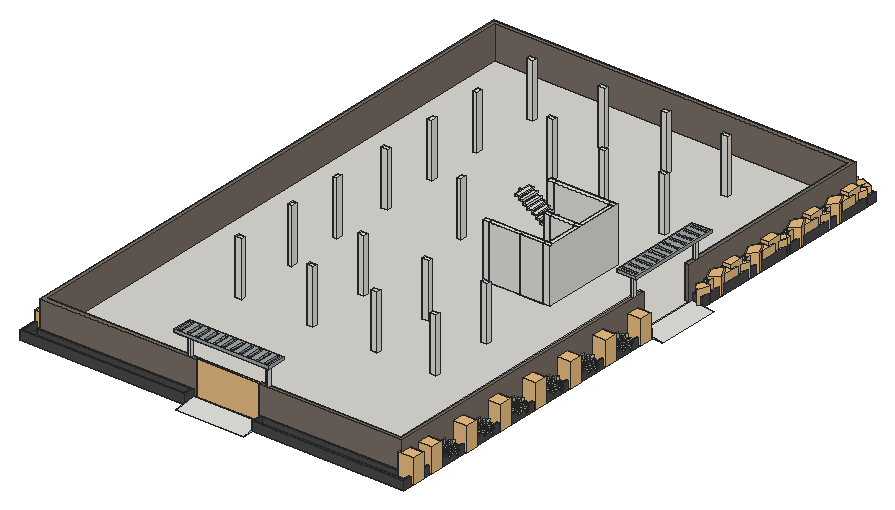
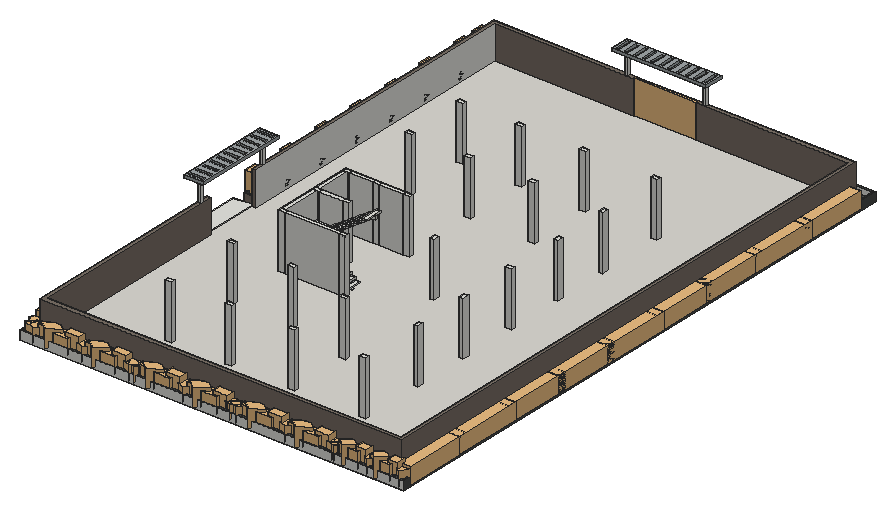
# SketchUp Ruby script. Lengths in inches.
U = 1.inch
M = Sketchup.active_model
def pt(a) = Geom::Point3d.new(a.map { |v| v * U })
def face(e, loops, mat)
  f = e.add_face(loops[0].map { |a| pt(a) })
  loops[1..].each { |l| e.add_face(l.map { |a| pt(a) }).erase! }
  f.material = f.back_material = mat if mat
  f
end
# faces: each face lists its corners as indices into pts; further lists are holes
def faces(e, pts, list, mat = nil) = list.each { |f| face(e, (f[0].is_a?(Array) ? f : [f]).map { |l| l.map { |i| pts[i] } }, mat) }
# xy, xz, yz: faces in a plane at the given z, y or x. An outline is a flat list of corners, or four numbers for a rectangle; further outlines are holes
def ring(l) = l.size == 4 ? [[l[0], l[1]], [l[2], l[1]], [l[2], l[3]], [l[0], l[3]]] : l.each_slice(2).to_a
def flat(e, list, mat, &to3) = list.each { |f| face(e, (f[0].is_a?(Array) ? f : [f]).map { |l| ring(l).map { |u, v| to3.(u, v) } }, mat) }
def xy(e, z, list, mat = nil) = flat(e, list, mat) { |x, y| [x, y, z] }
def xz(e, y, list, mat = nil) = flat(e, list, mat) { |x, z| [x, y, z] }
def yz(e, x, list, mat = nil) = flat(e, list, mat) { |y, z| [x, y, z] }
def lines(e, pts, list) = list.each { |a, b| e.add_line(pt(pts[a]), pt(pts[b])) }
# prism: a flat outline (further loops are holes) pulled along v
def prism(e, loops, v, mat = nil)
  f = face(e, loops, mat); d = Geom::Vector3d.new(v.map { |x| x * U })
  f.pushpull(f.normal.samedirection?(d) ? d.length : -d.length)
end
def box(e, o, s, mat = nil) = prism(e, [[o, [o[0] + s[0], o[1], o[2]], [o[0] + s[0], o[1] + s[1], o[2]], [o[0], o[1] + s[1], o[2]]]], [0, 0, s[2]], mat)
def at(x, y, z, deg = 0) = Geom::Transformation.translation(pt([x, y, z])) * Geom::Transformation.rotation(ORIGIN, Z_AXIS, deg.degrees)
def axes(o, x, y, z) = Geom::Transformation.new([*x, 0, *y, 0, *z, 0, *pt(o).to_a, 1])
def part(name) = M.definitions.add(name)
# library, detail: a bought-in or finely detailed component or shape, given as its bounding box
def library(name, o, s) = part(name).tap { |d| box(d.entities, o, s) }
def detail(e, o, s) = box(e.add_group.entities, o, s)
def put(e, d, t, mat = nil) = e.add_instance(d, t).tap { |i| i.material = mat if mat }
def group(e, t, mat = nil) = e.add_group.tap { |g| g.transformation = t; g.material = mat if mat }.entities
root = M.entities
M.materials.add("1484 AP 8289 COLD FLINT").color = [159, 165, 167]
M.materials.add("1488 AP 8285 MINESHAFT").color = [72, 74, 72]
M.materials.add("1495 AP 8294 DARK SHADOW").color = [102, 101, 98]
M.materials.add("Material__3").color = [95, 70, 46]
M.materials.add("StoneBricksSplitface001_4K").color = [121, 111, 102]
M.materials.add("[Terrazzo Tile Light]").color = [219, 217, 210]
M.materials.add("hymenocallis littoralis").color = [156, 172, 146]
c1 = part("1")
box(c1.entities,[0,0,0],[14,9,117])
c2 = part("Group\#131")
box(c2.entities,[0,0,0],[6,6,48])
c3 = library("Group\#239",[0,0,-0.25],[37,199,0.25])
c4 = part("21")
put(c4.entities,c2,at(18,15,0))
g1 = group(c4.entities,at(18,12,48),"1484 AP 8289 COLD FLINT")
xy(g1,0,[[-18,-12,24,192]],"1484 AP 8289 COLD FLINT")
xy(g1,6,[[[-18,-12,24,192],[-12,-6,18,0],[-12,12.6,18,18.6],[-12,31.2,18,37.2],[-12,49.8,18,55.8],[-12,68.4,18,74.4],[-12,87,18,93],[-12,105.6,18,111.6],[-12,124.2,18,130.2],[-12,142.8,18,148.8],[-12,161.4,18,167.4],[-12,180,18,186]]])
xz(g1,-12,[[-18,0,24,6]],"1484 AP 8289 COLD FLINT")
xz(g1,-6,[[-12,0,18,6]])
xz(g1,0,[[-12,0,18,6]])
xz(g1,12.6,[[-12,0,18,6]])
xz(g1,18.6,[[-12,0,18,6]])
xz(g1,31.2,[[-12,0,18,6]])
xz(g1,37.2,[[-12,0,18,6]])
xz(g1,49.8,[[-12,0,18,6]])
xz(g1,55.8,[[-12,0,18,6]])
xz(g1,68.4,[[-12,0,18,6]])
xz(g1,74.4,[[-12,0,18,6]])
xz(g1,87,[[-12,0,18,6]])
xz(g1,93,[[-12,0,18,6]])
xz(g1,105.6,[[-12,0,18,6]])
xz(g1,111.6,[[-12,0,18,6]])
xz(g1,124.2,[[-12,0,18,6]])
xz(g1,130.2,[[-12,0,18,6]])
xz(g1,142.8,[[-12,0,18,6]])
xz(g1,148.8,[[-12,0,18,6]])
xz(g1,161.4,[[-12,0,18,6]])
xz(g1,167.4,[[-12,0,18,6]])
xz(g1,180,[[-12,0,18,6]])
xz(g1,186,[[-12,0,18,6]])
xz(g1,192,[[-18,0,24,6]])
yz(g1,-18,[[-12,0,192,6]],"1484 AP 8289 COLD FLINT")
yz(g1,-12,[[-6,0,0,6],[12.6,0,18.6,6],[31.2,0,37.2,6],[49.8,0,55.8,6],[68.4,0,74.4,6],
  [87,0,93,6],[105.6,0,111.6,6],[124.2,0,130.2,6],[142.8,0,148.8,6],[161.4,0,167.4,6],
  [180,0,186,6]])
yz(g1,18,[[-6,0,0,6],[12.6,0,18.6,6],[31.2,0,37.2,6],[49.8,0,55.8,6],[68.4,0,74.4,6],
  [87,0,93,6],[105.6,0,111.6,6],[124.2,0,130.2,6],[142.8,0,148.8,6],[161.4,0,167.4,6],
  [180,0,186,6]])
yz(g1,24,[[-12,0,192,6]])
put(g1,c3,at(-15.5,-9.5,0))
g2 = group(g1,at(22,-10,0),"1495 AP 8294 DARK SHADOW")
xy(g2,-0.5,[[[-38,0,0,200],[-37.5,0.5,-0.5,199.5]]])
xz(g2,0,[[-38,-0.5,0,0]])
xz(g2,0.5,[[-37.5,-0.5,-0.5,0]])
xz(g2,199.5,[[-37.5,-0.5,-0.5,0]])
xz(g2,200,[[-38,-0.5,0,0]])
yz(g2,-38,[[0,-0.5,200,0]])
yz(g2,-37.5,[[0.5,-0.5,199.5,0]])
yz(g2,-0.5,[[0.5,-0.5,199.5,0]])
yz(g2,0,[[0,-0.5,200,0]])
put(c4.entities,c2,axes([18,189,0],[1,0,0],[0,-1,0],[0,0,1]))
c5 = library("Gate_Lasercut_10ftx6ft_Kalil",[-0.15,-3.25,-0.15],[120,5.625,60.3])
c6 = part("90")
box(c6.entities,[0,-39,3],[11,39,3])
c7 = part("Group\#94")
box(c7.entities,[-50,0,0],[50,9,117])
c8 = part("Group\#856")
xy(c8.entities,7.38,[[0,0,5.5,15.91]],"hymenocallis littoralis")
p = [[5.5,28.78,0],[5.5,26.79,3.44],[0,26.79,3.44],[0,28.78,0],[0,23.75,6],[5.5,23.75,6],
  [0,15.91,7.38],[5.5,15.91,7.38]]
faces(c8.entities,p,[[0,1,2,3],[4,2,1,5],[6,4,5,7]],"hymenocallis littoralis")
c9 = part("Group\#854")
xy(c9.entities,7.38,[[0,0,5.5,15.91],[0,15.91,5.5,23.87]],"hymenocallis littoralis")
p = [[5.5,31.07,4.3],[5.5,27.74,6.47],[0,27.74,6.47],[0,31.07,4.3],[0,23.87,7.38],[5.5,23.87,7.38]]
faces(c9.entities,p,[[0,1,2,3],[4,2,1,5]],"hymenocallis littoralis")
c10 = part("Group\#857")
xy(c10.entities,7.38,[[0,0,5.6,15.91]],"hymenocallis littoralis")
p = [[5.6,28.78,0],[5.6,26.79,3.44],[0,26.79,3.44],[0,28.78,0],[0,23.75,6],[5.6,23.75,6],
  [0,15.91,7.38],[5.6,15.91,7.38]]
faces(c10.entities,p,[[0,1,2,3],[4,2,1,5],[6,4,5,7]],"hymenocallis littoralis")
c11 = part("Group\#855")
put(c11.entities,c9,axes([6.09,8.57,-0.52],[0.446,0.85617,0.26089],[-0.18444,-0.19731,0.96283],[0.87582,-0.47754,0.0699]))
put(c11.entities,c9,axes([6.29,7.28,-1.71],[0.37058,0.92707,-0.05667],[-0.32382,0.19004,0.99128],[0.87712,-0.32925,0.34964]))
put(c11.entities,c9,axes([11.04,16.14,-0.7],[1,0,0],[0,0.16628,1.02662],[0,-1.18456,0.19186]))
c12 = part("Group\#860")
put(c12.entities,c8,axes([24.57,32.05,-1.76],[0.9552,-0.22102,-0.19681],[0.4036,0.95545,0.88585],[-0.00568,-0.67859,0.7345]))
put(c12.entities,c8,axes([23.95,29.24,-2.4],[0,1,0],[-0.76041,0,0.64945],[0.64945,0,0.76041]))
put(c12.entities,c8,axes([24.22,24.72,-0.48],[-0.70711,0.70711,0],[-0.32757,-0.32757,0.80237],[0.61237,0.61237,0.5]))
put(c12.entities,c9,axes([20.66,37.22,-0.63],[1.12361,0.03262,0.39091],[-0.43499,0.29739,0.78777],[0.09852,-1.27434,0.37535]))
put(c12.entities,c8,axes([28.75,24.45,-2.4],[-1,0,0],[0,-0.76041,0.64945],[0,0.64945,0.76041]))
put(c12.entities,c10,axes([30.4,30.98,-3.7],[0.65676,-0.72002,0.22414],[0.55667,0.66341,0.5],[-0.50871,-0.20361,0.83652]))
put(c12.entities,c10,axes([32.41,29.61,-3.7],[0.04029,-0.97372,0.22414],[0.85287,0.15038,0.5],[-0.52057,0.17102,0.83652]))
put(c12.entities,c8,axes([31.89,25.85,-1.76],[-0.92056,0.33739,-0.19681],[-0.5186,-0.89824,0.88585],[0.08952,0.67268,0.7345]))
put(c12.entities,c8,axes([25.55,34.78,-0.48],[0.86603,0.5,0],[-0.25,0.43301,0.86603],[0.43301,-0.75,0.5]))
put(c12.entities,c10,axes([20.4,16.9375,-8.07],[-0.70711,0.70711,0],[-0.35754,-0.35754,0.65422],[1.3987,1.3987,1.52882]))
put(c12.entities,c8,axes([32.86,34.14,-0.48],[0.76604,-0.64279,0],[0.32139,0.38302,0.86603],[-0.55667,-0.66341,0.5]))
put(c12.entities,c8,axes([27.15,34.7,-0.1],[0.82472,-0.17528,-0.53769],[0.53769,0.53769,0.64945],[0.17528,-0.82472,0.53769]))
put(c12.entities,c8,axes([33.58,28.77,-2.4],[0,-1,0],[0.76041,0,0.64945],[-0.64945,0,0.76041]))
put(c12.entities,c8,axes([26.43,23.87,-2.81],[-0.75126,0.04415,0.65853],[0.53769,-0.53769,0.64945],[0.38276,0.84199,0.3802]))
put(c12.entities,c8,axes([28.78,23.98,-2.4],[-1,0,0],[0,-0.76041,0.64945],[0,0.64945,0.76041]))
put(c12.entities,c8,axes([25.39,25.38,-2.4],[-0.70711,0.70711,0],[-0.53769,-0.53769,0.64945],[0.45923,0.45923,0.76041]))
put(c12.entities,c8,axes([27.32,21.63,-0.1],[-0.45923,0.70711,-0.53769],[-0.76041,0,0.64945],[0.45923,0.70711,0.53769]))
put(c12.entities,c8,axes([25.17,27.625,-1.76],[0.56416,0.80187,-0.19681],[-0.66673,0.66673,0.80532],[0.62659,-0.26057,0.7345]))
put(c12.entities,c10,axes([27.59,27.04,-3.96],[-0.8993,-0.06127,0.43301],[0.2962,-0.8138,0.5],[0.32175,0.57791,0.75]))
put(c12.entities,c10,axes([26.98,24.5,-3.18],[-0.5,0.86603,0],[-0.75,-0.43301,0.5],[0.43301,0.25,0.86603]))
put(c12.entities,c10,axes([24.55,27.74,-3.7],[0.29517,0.92878,0.22414],[-0.85287,0.15038,0.5],[0.43068,-0.33875,0.83652]))
put(c12.entities,c10,axes([24.26,29.8,-3.18],[0.76604,0.64279,0],[-0.47317,0.5639,0.425],[0.32139,-0.38302,0.86603]))
put(c12.entities,c10,axes([25.98,32.46,-3.18],[1,0,0],[0,0.86603,0.5],[0,-0.5,0.86603]))
put(c12.entities,c8,axes([28.78,33.57,-2.4],[1,0,0],[0,0.76041,0.64945],[0,-0.64945,0.76041]))
put(c12.entities,c11,at(14.99,21.38,2.5))
put(c12.entities,c9,axes([34.63,26.34,-1.46],[-0.70089,-0.70877,0.07994],[0.4756,-0.38088,0.79293],[-0.53156,0.59378,0.60405]))
put(c12.entities,c9,axes([28.14,16.92,1.8125],[-1.19719,0.6912,0],[-0.09607,-0.16641,0.94244],[0.68444,1.18549,0.17613]))
put(c12.entities,c9,axes([31.5625,35.84,0.97],[0.66765,-1.1564,0.35779],[0.04445,0.30732,0.91033],[-1.20828,-0.64496,0.17012]))
put(c12.entities,c9,axes([38.94,22.51,0.89],[-0.97932,-0.67164,-0.05202],[0.27787,-0.41401,0.90999],[-0.85985,0.93577,0.32097]))
put(c12.entities,c9,axes([38.44,21.09,1.98],[-1.02864,-0.54856,0.2395],[0.33481,0.06999,0.88388],[-0.77261,1.08328,0.06417]))
put(c12.entities,c10,axes([35.02,30.51,-1.3],[-0.17365,-0.98481,0],[0.60224,-0.10619,0.79122],[-0.7792,0.13739,0.61153]))
put(c12.entities,c10,axes([29.41,22.33,-1.3],[-0.93969,0.34202,0],[-0.20915,-0.57465,0.79122],[0.27061,0.74351,0.61153]))
put(c12.entities,c9,axes([19.64,36,-1.62],[1.18194,0.09546,0.08234],[-0.14377,0.68823,0.76313],[0.21457,-1.1326,0.62386]))
put(c12.entities,c10,axes([24.25,24.14,-1.3],[-0.34202,0.93969,0],[-0.57465,-0.20915,0.79122],[0.74351,0.27061,0.61153]))
put(c12.entities,c10,axes([25.98,34.61,-1.3],[1,0,0],[0,0.61153,0.79122],[0,-0.79122,0.61153]))
put(c12.entities,c10,axes([31.16,34.41,-1.64],[0.56518,-0.80224,-0.19234],[0.73413,0.34233,0.72935],[-0.47639,-0.50772,0.71782]))
put(c12.entities,c10,axes([40.52,26.84,-5.82],[-0.42262,-0.90631,0],[0.48019,-0.22391,0.68552],[-1.43418,0.66877,1.22305]))
put(c12.entities,c8,axes([29.86,38.42,-1.01],[0.89064,-0.37013,0.26413],[-0.03924,0.63286,1.01918],[-0.45353,-0.76487,0.45748]))
put(c12.entities,c8,axes([29.34,22.4,-0.48],[-0.99619,-0.08716,0],[0.04358,-0.4981,0.86603],[-0.07548,0.86273,0.5]))
c13 = part("Group\#858")
xz(c13.entities,10.07,[[9.07,0,10.07,31.01],[0,31.01,0,45.12,20.13,45.12,20.13,31.01,10.07,31.01,10.07,32.58,9.07,32.58,9.07,31.01]],"hymenocallis littoralis")
yz(c13.entities,10.07,[[0,31.01,20.13,45.12]],"hymenocallis littoralis")
p = [[9.57,9.2,0],[10.07,10.07,0],[10.07,10.07,31.01],[10.07,10.07,32.58],[9.57,9.2,32.58]]
faces(c13.entities,p,[[0,1,2,3,4]],"hymenocallis littoralis")
c14 = part("cây lá nắng")
put(c14.entities,c12,axes([49.26,-2.75,0],[0.63109,0.63109,0],[-0.63109,0.63109,0],[0,0,0.935]))
g3 = group(c14.entities,at(26.6,-8.68,0))
put(g3,c8,axes([-4.72,35.73,-1.65],[0.74231,0.46334,-0.18402],[-0.34827,0.85768,0.82827],[0.42467,-0.43184,0.68675]))
put(g3,c8,axes([-3.34,33.57,-2.24],[-0.63109,0.63109,0],[-0.47989,-0.47989,0.60723],[0.40986,0.40986,0.71098]))
put(g3,c8,axes([-0.3125,30.89,-0.45],[-0.8925,0,0],[0,-0.41345,0.75022],[0,0.77293,0.4675]))
put(g3,c9,axes([-10.79,39.66,-0.59],[0.68852,0.72969,0.3655],[-0.4622,-0.08684,0.73657],[0.86641,-0.74205,0.35095]))
put(g3,c8,axes([2.71,33.57,-2.24],[-0.63109,-0.63109,0],[0.47989,-0.47989,0.60723],[-0.40986,0.40986,0.71098]))
put(g3,c10,axes([-0.37,38.74,-3.46],[0.86887,-0.03992,0.20957],[-0.06737,0.76999,0.4675],[-0.19255,-0.44954,0.78214]))
put(g3,c10,axes([1.76,39.14,-3.46],[0.63993,-0.58908,0.20957],[0.44333,0.63315,0.4675],[-0.43646,-0.2206,0.78214]))
put(g3,c8,axes([3.81,36.4375,-1.65],[-0.79389,-0.36803,-0.18402],[0.23959,-0.89415,0.82827],[-0.36803,0.48102,0.68675]))
put(g3,c8,axes([-5.83,38.07,-0.45],[0.231,0.86209,0],[-0.43104,0.1155,0.80973],[0.74659,-0.20005,0.4675]))
put(g3,c10,axes([2.18,23.5625,-7.55],[-0.8925,0,0],[0,-0.45128,0.6117],[0,1.76542,1.42944]))
put(g3,c8,axes([-0.8125,42.28,-0.45],[0.8891,0.07779,0],[-0.03889,0.44455,0.80973],[0.06737,-0.76999,0.4675]))
put(g3,c8,axes([-4.76,39.03,-0.09],[0.63109,0.40986,-0.50274],[0,0.67866,0.60723],[0.63109,-0.40986,0.50274]))
put(g3,c8,axes([3.03,39.35,-2.24],[0.63109,-0.63109,0],[0.47989,0.47989,0.60723],[-0.40986,-0.40986,0.71098]))
put(g3,c8,axes([1.61,31.74,-2.625],[-0.50198,-0.44625,0.61573],[0.67866,0,0.60723],[-0.28982,0.77293,0.35549]))
put(g3,c8,axes([3.03,33.3,-2.24],[-0.63109,-0.63109,0],[0.47989,-0.47989,0.60723],[-0.40986,0.40986,0.71098]))
put(g3,c8,axes([0.01,32.04,-2.24],[-0.8925,0,0],[0,-0.67866,0.60723],[0,0.57963,0.71098]))
put(g3,c8,axes([3.59,30.89,-0.09],[-0.73607,0.15643,-0.50274],[-0.47989,-0.47989,0.60723],[-0.15643,0.73607,0.50274]))
put(g3,c8,axes([-1.55,33.32,-1.65],[-0.15002,0.86209,-0.18402],[-0.84154,0,0.75297],[0.55988,0.231,0.68675]))
put(g3,c10,axes([0.35,34.48,-3.71],[-0.52887,-0.60621,0.40487],[0.70051,-0.32665,0.4675],[-0.16166,0.56777,0.70125]))
put(g3,c10,axes([2.61,39.13,-1.74],[-0.86209,0.231,0],[-0.23031,-0.85954,0.15531],[0.03162,0.11799,0.91645]))
put(g3,c10,axes([-2.02,33,-3.46],[-0.39986,0.77243,0.20957],[-0.63315,-0.44333,0.4675],[0.48558,0.05802,0.78214]))
put(g3,c10,axes([-3.49,34.12,-2.97],[0.07779,0.8891,0],[-0.65449,0.05726,0.39737],[0.44455,-0.03889,0.80973]))
put(g3,c10,axes([-4.09,36.88,-2.97],[0.63109,0.63109,0],[-0.54654,0.54654,0.4675],[0.31555,-0.31555,0.80973]))
put(g3,c8,axes([-3.02,39.35,-2.24],[0.63109,0.63109,0],[-0.47989,0.47989,0.60723],[0.40986,-0.40986,0.71098]))
put(g3,c11,axes([-4.03,22.95,2.33],[0.63109,0.63109,0],[-0.63109,0.63109,0],[0,0,0.935]))
put(g3,c9,axes([5.24,38.48,-1.37],[0.00497,-0.88963,0.07474],[0.54052,0.05978,0.74139],[-0.71019,0.03927,0.56479]))
put(g3,c9,axes([7.08,28.4375,1.7],[-1.19175,-0.31933,0],[0.04439,-0.16565,0.88118],[-0.31621,1.1801,0.16468]))
put(g3,c9,axes([-2.7,42.54,0.91],[1.15114,-0.30845,0.33454],[-0.1659,0.22199,0.85115],[-0.3555,-1.16957,0.15907]))
put(g3,c9,axes([10.37,38.78,0.83],[-0.19417,-1.04191,-0.04864],[0.43664,-0.08592,0.85084],[-1.1332,0.04791,0.30011]))
put(g3,c9,axes([10.95,37.5625,1.85],[-0.30298,-0.99536,0.22393],[0.16713,0.25547,0.82643],[-1.17124,0.19607,0.06]))
put(g3,c10,axes([2.84,41.36,-1.22],[0.51192,-0.73109,0],[0.44708,0.31305,0.73979],[-0.57846,-0.40504,0.57178]))
put(g3,c10,axes([4.47,32.65,-1.22],[-0.80888,-0.37719,0],[0.23066,-0.49465,0.73979],[-0.29844,0.64,0.57178]))
put(g3,c9,axes([-10.32,35.12,-1.51],[0.68567,0.80616,0.07699],[-0.52507,0.3436,0.71352],[0.85019,-0.57936,0.58331]))
put(g3,c10,axes([0.07,30.54,-1.22],[-0.80888,0.37719,0],[-0.23066,-0.49465,0.73979],[0.29844,0.64,0.57178]))
put(g3,c10,axes([-5.45,38.24,-1.22],[0.63109,0.63109,0],[-0.38593,0.38593,0.73979],[0.49934,-0.49934,0.57178]))
put(g3,c10,axes([-2.05,41.38,-1.53],[0.86296,-0.14961,-0.17984],[0.24726,0.67935,0.68194],[0.01977,-0.62107,0.67116]))
put(g3,c10,axes([8.63,42.51,-5.4375],[0.30525,-0.83868,0],[0.44435,0.16173,0.64096],[-1.32716,-0.48305,1.14356]))
put(g3,c8,axes([-5.4,43.09,-0.94],[0.79566,0.32849,0.24696],[-0.42416,0.37462,0.95293],[0.19648,-0.76892,0.42774]))
put(g3,c8,axes([4.38,32.65,-0.45],[-0.57369,-0.68369,0],[0.34185,-0.28684,0.80973],[-0.5921,0.49683,0.4675]))
put(g3,c10,axes([-2,33.84,-0.15],[-0.24601,0.85793,0],[-0.85539,-0.24528,0.15531],[0.11742,0.03367,0.91645]))
put(g3,c10,axes([0.17,30.83,-4.47],[-0.24601,0.85793,0],[-0.85539,-0.24528,0.15531],[0.11742,0.03367,0.91645]))
put(g3,c10,axes([-1.97,32.18,-4.47],[0.58524,0.67383,0],[-0.67184,0.58351,0.15531],[0.09222,-0.0801,0.91645]))
put(g3,c10,axes([-2,34.71,-4.47],[0.88392,-0.12346,0],[0.12309,0.88131,0.15531],[-0.0169,-0.12098,0.91645]))
put(g3,c10,axes([0.11,36.12,-4.47],[0.37822,-0.8084,0],[0.80601,0.37711,0.15531],[-0.11064,-0.05177,0.91645]))
put(c14.entities,c13,axes([29.71,14.29,6.94],[0.425,0.73612,0],[-0.6771,0.39092,-0.33349],[-0.26859,0.15507,0.72712]))
put(c14.entities,c13,axes([42.0625,26.12,6.94],[0.85,0,0],[0,0.78185,-0.33349],[0,0.33349,0.78185]))
put(c14.entities,c12,axes([7.3125,23.0625,0],[0.8925,0,0],[0,0.8925,0],[0,0,0.935]))
put(c14.entities,c13,axes([24.4375,40.23,2.05],[0.85,0,0],[0,0.85,0],[0,0,0.85]))
c15 = library("Areca palm plant",[0,0,0],[49.1,36.6,54.46])
c16 = library("Group\#217",[-84.69,-90.07,-0.36],[176.51,175.13,171.4])
c17 = library("Group20\#1",[-20.81,-17.08,3.79],[39.86,39.43,37.51])
c18 = library("Group\#218",[-7.34,-1.2,0],[38.67,35.81,49.04])
c19 = library("Group38\#2",[14.01,28.44,-23.43],[18.58,18.32,38.89])
c20 = part("PLANTS\#1")
put(c20.entities,c15,axes([38.49,169.84,6.02],[0.45017,-0.56191,0],[0.66137,0.52986,0],[0,0,0.72]))
put(c20.entities,c15,axes([38.49,68.02,6.02],[0.45017,-0.56191,0],[0.66137,0.52986,0],[0,0,0.72]))
put(c20.entities,c16,axes([59.61,184.54,5.99],[-0.04961,-0.08593,0],[0.08593,-0.04961,0],[0,0,0.10522]))
put(c20.entities,c16,axes([59.61,204.61,5.99],[-0.04961,-0.08593,0],[0.08593,-0.04961,0],[0,0,0.10522]))
put(c20.entities,c16,axes([59.61,157.29,5.99],[-0.04961,-0.08593,0],[0.08593,-0.04961,0],[0,0,0.10522]))
put(c20.entities,c17,axes([63.65,91.4,4.71],[0,0.85,0],[-0.85,0,0],[0,0,0.85]))
put(c20.entities,c18,axes([69.62,101.34,7.93],[0,0.79,0],[-0.79,0,0],[0,0,0.79]))
put(c20.entities,c19,axes([40.58,10.27,28.11],[0.8848,0,0],[0,0.94674,0],[0,0,0.85826]))
put(c20.entities,c16,axes([59.61,55.48,5.99],[-0.04961,-0.08593,0],[0.08593,-0.04961,0],[0,0,0.10522]))
put(c20.entities,c16,axes([59.61,82.73,5.99],[-0.04961,-0.08593,0],[0.08593,-0.04961,0],[0,0,0.10522]))
put(c20.entities,c16,axes([61.875,132.66,6.01],[-0.08133,-0.14087,0],[0.14087,-0.08133,0],[0,0,0.1725]))
put(c20.entities,c16,axes([59.61,102.79,5.99],[-0.04961,-0.08593,0],[0.08593,-0.04961,0],[0,0,0.10522]))
put(c20.entities,c16,axes([61.875,27.22,6.01],[-0.08133,-0.14087,0],[0.14087,-0.08133,0],[0,0,0.1725]))
put(c20.entities,c16,axes([61.875,234.47,6.01],[-0.08133,-0.14087,0],[0.14087,-0.08133,0],[0,0,0.1725]))
put(c20.entities,c18,axes([69.62,203.15,7.93],[0,0.79,0],[-0.79,0,0],[0,0,0.79]))
put(c20.entities,c17,axes([63.65,193.21,4.71],[0,0.85,0],[-0.85,0,0],[0,0,0.85]))
put(c20.entities,c19,axes([40.58,112.08,28.11],[0.8848,0,0],[0,0.94674,0],[0,0,0.85826]))
g4 = group(c20.entities,at(44.68,11.43,-0.0625))
xy(g4,7,[[6,5,30,229.8]],"Material__3")
c21 = library("Living wall panel",[0,-0.29,-1.5625],[26.4375,4.09,16.41])
c22 = part("Plant Wall Garden (2)")
put(c22.entities,c21,axes([2954.1,2786.73,482.59],[-5.6832,0,0],[0,-8.46797,0],[0,0,6.64934]))
put(c22.entities,c21,axes([2820.97,2786.73,482.59],[-5.6832,0,0],[0,-8.46797,0],[0,0,6.64934]))
put(c22.entities,c21,axes([2687.85,2786.73,482.59],[-5.6832,0,0],[0,-8.46797,0],[0,0,6.64934]))
put(c22.entities,c21,axes([2554.72,2786.73,482.59],[-5.6832,0,0],[0,-8.46797,0],[0,0,6.64934]))
put(c22.entities,c21,axes([2421.6,2786.73,482.59],[-5.6832,0,0],[0,-8.46797,0],[0,0,6.64934]))
put(c22.entities,c21,axes([2288.47,2786.73,482.59],[-5.6832,0,0],[0,-8.46797,0],[0,0,6.64934]))
put(c22.entities,c21,axes([2155.35,2786.73,482.59],[-5.6832,0,0],[0,-8.46797,0],[0,0,6.64934]))
put(c22.entities,c21,axes([2022.22,2786.73,482.59],[-5.6832,0,0],[0,-8.46797,0],[0,0,6.64934]))
put(c22.entities,c21,axes([1889.1,2786.73,482.59],[-5.6832,0,0],[0,-8.46797,0],[0,0,6.64934]))
c23 = library("Plant (3)",[-15.5,2.64,0],[117.71,96.38,184.75])
g5 = group(root,at(144,357.97,0))
xy(g5,-6,[[-144,-333.97,-144,939,685.5,939,685.5,472.41,661.5,472.41,661.5,915,-120,915,-120,-310,211.65,-310,211.65,-333.97],[357.83,-333.97,357.83,-310,661.5,-310,661.5,334.62,685.5,334.62,685.5,-333.97]])
xy(g5,-6,[[-120,-310,661.5,915]],"[Terrazzo Tile Light]")
xy(g5,-1.61,[[-141,-330.97,208.65,-330.97,208.65,-313,-123,-313,-123,918,664.5,918,664.5,475.41,682.5,475.41,682.5,936,-141,936],[360.83,-330.97,682.5,-330.97,682.5,331.62,664.5,331.62,664.5,-313,360.83,-313]],"1488 AP 8285 MINESHAFT")
xy(g5,0,[[217.92,-310,352.5,-310,352.5,-301,652.5,-301,652.5,343.71,661.5,343.71,661.5,463.71,652.5,463.71,652.5,906,-111,906,-111,-301,217.92,-301]],"[Terrazzo Tile Light]")
xy(g5,13.39,[[[-144,-333.97,211.65,-333.97,211.65,-310,-120,-310,-120,915,661.5,915,661.5,472.41,685.5,472.41,685.5,939,-144,939],[-141,-330.97,-141,936,682.5,936,682.5,475.41,664.5,475.41,664.5,918,-123,918,-123,-313,208.65,-313,208.65,-330.97]],[[357.83,-333.97,685.5,-333.97,685.5,334.62,661.5,334.62,661.5,-310,357.83,-310],[360.83,-330.97,360.83,-313,664.5,-313,664.5,331.62,682.5,331.62,682.5,-330.97]]],"1488 AP 8285 MINESHAFT")
xy(g5,72,[[-120,-310,217.92,-310,217.92,-301,-111,-301,-111,906,652.5,906,652.5,463.71,661.5,463.71,661.5,915,-120,915],[352.5,-310,661.5,-310,661.5,343.71,652.5,343.71,652.5,-301,352.5,-301]],"StoneBricksSplitface001_4K")
xz(g5,-333.97,[[-144,-6,211.65,13.39],[357.83,-6,685.5,13.39]],"1488 AP 8285 MINESHAFT")
xz(g5,-330.97,[[-141,-1.61,208.65,13.39]])
xz(g5,-330.97,[[360.83,-1.61,682.5,13.39]],"1488 AP 8285 MINESHAFT")
xz(g5,-313,[[-123,-1.61,208.65,13.39],[360.83,-1.61,664.5,13.39]],"1488 AP 8285 MINESHAFT")
xz(g5,-310,[[-120,-6,211.65,13.39],[357.83,-6,661.5,13.39]])
xz(g5,-310,[[211.65,0,217.92,0,217.92,72,-120,72,-120,13.39,211.65,13.39],[352.5,0,357.83,0,357.83,13.39,661.5,13.39,661.5,72,352.5,72]],"StoneBricksSplitface001_4K")
xz(g5,-301,[[-111,0,217.92,72],[352.5,0,652.5,72]],"StoneBricksSplitface001_4K")
xz(g5,331.62,[[664.5,-1.61,682.5,13.39]],"1488 AP 8285 MINESHAFT")
xz(g5,334.62,[[661.5,-6,685.5,13.39]],"StoneBricksSplitface001_4K")
xz(g5,343.71,[[652.5,0,661.5,72]],"StoneBricksSplitface001_4K")
xz(g5,463.71,[[652.5,0,661.5,72]],"StoneBricksSplitface001_4K")
xz(g5,472.41,[[661.5,-6,685.5,13.39]],"1488 AP 8285 MINESHAFT")
xz(g5,475.41,[[664.5,-1.61,682.5,13.39]],"1488 AP 8285 MINESHAFT")
xz(g5,906,[[-111,0,652.5,72]],"StoneBricksSplitface001_4K")
xz(g5,915,[[-120,-6,661.5,13.39]])
xz(g5,915,[[-120,13.39,661.5,72]],"StoneBricksSplitface001_4K")
xz(g5,918,[[-123,-1.61,664.5,13.39]])
xz(g5,936,[[-141,-1.61,682.5,13.39]],"StoneBricksSplitface001_4K")
xz(g5,939,[[-144,-6,685.5,13.39]])
yz(g5,-144,[[-333.97,-6,939,13.39]],"1488 AP 8285 MINESHAFT")
yz(g5,-141,[[-330.97,-1.61,936,13.39]],"1488 AP 8285 MINESHAFT")
yz(g5,-123,[[-313,-1.61,918,13.39]],"1488 AP 8285 MINESHAFT")
yz(g5,-120,[[-310,-6,915,13.39]])
yz(g5,-120,[[-310,13.39,915,72]],"StoneBricksSplitface001_4K")
yz(g5,-111,[[-301,0,906,72]],"StoneBricksSplitface001_4K")
yz(g5,208.65,[[-330.97,-1.61,-313,13.39]],"1488 AP 8285 MINESHAFT")
yz(g5,211.65,[[-333.97,-6,-310,13.39]],"1488 AP 8285 MINESHAFT")
yz(g5,217.92,[[-310,0,-301,72]],"StoneBricksSplitface001_4K")
yz(g5,352.5,[[-310,0,-301,72]],"StoneBricksSplitface001_4K")
yz(g5,357.83,[[-333.97,-6,-310,13.39]],"1488 AP 8285 MINESHAFT")
yz(g5,360.83,[[-330.97,-1.61,-313,13.39]],"1488 AP 8285 MINESHAFT")
yz(g5,652.5,[[-301,0,343.71,72]])
yz(g5,652.5,[[463.71,0,906,72]],"StoneBricksSplitface001_4K")
yz(g5,661.5,[[-310,-6,334.62,13.39],[472.41,-6,915,13.39]])
yz(g5,661.5,[[334.62,-6,343.71,-6,343.71,72,-310,72,-310,13.39,334.62,13.39],[464.08,-6,472.41,-6,472.41,13.39,915,13.39,915,72,463.71,72,463.71,0,464.08,0]],"StoneBricksSplitface001_4K")
yz(g5,664.5,[[-313,-1.61,331.62,13.39],[475.41,-1.61,918,13.39]],"1488 AP 8285 MINESHAFT")
yz(g5,682.5,[[475.41,-1.61,936,13.39]])
yz(g5,682.5,[[-330.97,-1.61,331.62,13.39]],"1488 AP 8285 MINESHAFT")
yz(g5,685.5,[[-333.97,-6,334.62,13.39],[472.41,-6,939,13.39]],"1488 AP 8285 MINESHAFT")
put(g5,c1,at(54,0,0))
put(g5,c1,at(228,390.5,0,90))
put(g5,c1,at(63,141,0,90))
put(g5,c1,at(63,263,0,90))
put(g5,c1,at(54,393,0))
put(g5,c1,at(473.5,618,0))
put(g5,c1,at(208,138,0))
put(g5,c1,at(208,648,0))
put(g5,c1,at(473.5,786,0))
put(g5,c1,at(54,786,0))
put(g5,c1,at(473.5,0,0))
put(g5,c1,at(63,640,0,90))
put(g5,c1,at(409.5,387,0))
put(g5,c1,at(473.5,306,0))
put(g5,c1,at(343.5,480,0))
put(g5,c1,at(409.5,306,0))
put(g5,c1,at(208,0,0))
put(g5,c1,at(473.5,138,0))
put(g5,c1,at(343.5,786,0))
put(g5,c1,at(473.5,480,0))
put(g5,c1,at(473.5,387,0))
put(g5,c1,at(343.5,618,0))
put(g5,c1,at(346.5,138,0))
put(g5,c1,at(343.5,306,0))
put(g5,c1,at(346.5,0,0))
put(g5,c1,at(208,786,0))
put(g5,c1,at(63,518,0,90))
put(g5,c4,at(636,301.71,72))
put(g5,c4,at(183.02,-284.5,72,-90))
put(g5,c5,axes([217.94,-305.63,0.03],[1.12273,0,0],[0,-1,0],[0,0,1.19652]))
g6 = group(g5,at(349.5,396,0))
g7 = group(g6,at(90,39,60))
p = [[-2.14,-17.5,-4.57],[-2.14,-21.5,-4.57]]
lines(g7,p,[[0,1]])
put(g7,c6,axes([0,-39,0],[-0.81818,0,0],[0,-1,0],[0,0,1]))
put(g7,c6,axes([-63,-39,42],[-0.81818,0,0],[0,-1,0],[0,0,1]))
put(g7,c6,axes([-72,-39,48],[-0.81818,0,0],[0,-1,0],[0,0,1]))
put(g7,c6,axes([-9,-39,6],[-0.81818,0,0],[0,-1,0],[0,0,1]))
put(g7,c6,axes([-18,-39,12],[-0.81818,0,0],[0,-1,0],[0,0,1]))
put(g7,c6,axes([-27,-39,18],[-0.81818,0,0],[0,-1,0],[0,0,1]))
put(g7,c6,axes([-45,-39,30],[-0.81818,0,0],[0,-1,0],[0,0,1]))
put(g7,c6,axes([-81,-39,54],[-0.81818,0,0],[0,-1,0],[0,0,1]))
put(g7,c6,axes([-54,-39,36],[-0.81818,0,0],[0,-1,0],[0,0,1]))
put(g7,c6,axes([-36,-39,24],[-0.81818,0,0],[0,-1,0],[0,0,1]))
put(g7,c6,axes([-90,-39,60],[-0.81818,0,0],[0,-1,0],[0,0,1]))
g8 = group(g7,at(39,27.5,-59.5,180))
xy(g8,-4.5,[[121.99,0,129,4]])
xy(g8,-0.5,[[124.5,0,129,4]])
xy(g8,50.5,[[[0,0,0,4,7.52,4,7.52,45,0,45,0,49,42.08,49,42.08,45,31.52,45,31.52,4,42.5625,4,42.5625,0],[11.52,4,27.52,45]]])
xy(g8,53.5,[[7.52,4,11.52,4,11.52,45,27.52,45,27.52,4,31.52,4,31.52,45,39.05,45,39.05,49,0,49,0,45,7.52,45]])
xy(g8,53.52,[[0,0,39,4]])
xy(g8,56.5,[[39,0,42,4]])
xy(g8,57.92,[[39.05,45,41.14,49]])
xy(g8,119.5,[[138,45,144,49]])
xy(g8,125.5,[[138,45,144,49]])
xz(g8,0,[[121.99,-4.5,129,-4.5,129,-0.5,124.5,-0.5,42,54.5,42,56.5,39,56.5,39,53.52,0,53.52,0,50.5,42.5625,50.5,42.5625,50.52,121.99,-1.85]])
xz(g8,4,[[121.99,-4.5,121.99,-1.85,42.5625,50.52,42.5625,50.5,31.52,50.5,31.52,53.5,27.52,53.5,27.52,50.5,11.52,50.5,11.52,53.5,7.52,53.5,7.52,50.5,0,50.5,0,53.52,39,53.52,39,56.5,42,56.5,42,54.5,124.5,-0.5,129,-0.5,129,-4.5]])
xz(g8,45,[[0,50.5,7.52,53.5],[11.52,50.5,27.52,53.5],[31.52,50.5,42.08,50.5,42.08,55.54,138,119.5,144,119.5,144,125.5,138,125.5,138,122.5,129,116.5,41.14,57.92,39.05,57.92,39.05,53.5,31.52,53.5]])
xz(g8,49,[[0,50.5,0,53.5,39.05,53.5,39.05,57.92,41.14,57.92,129,116.5,138,122.5,138,125.5,144,125.5,144,119.5,138,119.5,42.08,55.54,42.08,50.5]])
yz(g8,0,[[0,50.5,4,53.52],[45,50.5,49,53.5]])
yz(g8,7.52,[[4,50.5,45,53.5]])
yz(g8,11.52,[[4,50.5,45,53.5]])
yz(g8,27.52,[[4,50.5,45,53.5]])
yz(g8,31.52,[[4,50.5,45,53.5]])
yz(g8,39,[[0,53.52,4,56.5]])
yz(g8,39.05,[[45,53.5,49,57.92]])
yz(g8,42,[[0,54.5,4,56.5]])
yz(g8,42.08,[[45,50.5,49,55.54]])
yz(g8,42.5625,[[0,50.5,4,50.52]])
yz(g8,121.99,[[0,-4.5,4,-1.85]])
yz(g8,129,[[0,-4.5,4,-0.5]])
yz(g8,138,[[45,122.5,49,125.5]])
yz(g8,144,[[45,119.5,49,125.5]])
p = [[42.5625,4,50.52],[121.99,4,-1.85],[121.99,0,-1.85],[42.5625,0,50.52],[124.5,4,-0.5],[42,4,54.5],
  [42,0,54.5],[124.5,0,-0.5],[138,49,119.5],[138,45,119.5],[42.08,45,55.54],[42.08,49,55.54],
  [129,49,116.5],[41.14,49,57.92],[41.14,45,57.92],[129,45,116.5],[138,49,122.5],[138,45,122.5],
  [124.99,4,-0.83],[124.99,0,-0.83]]
faces(g8,p,[[0,1,2,3],[4,5,6,7],[8,9,10,11],[12,13,14,15],[16,12,15,17]])
lines(g8,p,[[18,19]])
g9 = group(g6,at(0,45,0))
put(g9,c6,axes([0,39,0],[0.81818,0,0],[0,1,0],[0,0,1]))
put(g9,c6,axes([63,39,42],[0.81818,0,0],[0,1,0],[0,0,1]))
put(g9,c6,axes([72,39,48],[0.81818,0,0],[0,1,0],[0,0,1]))
put(g9,c6,axes([9,39,6],[0.81818,0,0],[0,1,0],[0,0,1]))
put(g9,c6,axes([18,39,12],[0.81818,0,0],[0,1,0],[0,0,1]))
put(g9,c6,axes([27,39,18],[0.81818,0,0],[0,1,0],[0,0,1]))
put(g9,c6,axes([45,39,30],[0.81818,0,0],[0,1,0],[0,0,1]))
put(g9,c6,axes([81,39,54],[0.81818,0,0],[0,1,0],[0,0,1]))
put(g9,c6,axes([54,39,36],[0.81818,0,0],[0,1,0],[0,0,1]))
put(g9,c6,axes([36,39,24],[0.81818,0,0],[0,1,0],[0,0,1]))
g10 = group(g6,at(90,0,54))
box(g10,[0,0,0],[39,84,6])
g11 = group(g5,at(478.5,480,54))
box(g11,[0,-84,-54],[9,84,117])
g12 = group(g5,at(478.5,387,54))
box(g12,[0,-72,-54],[9,72,117])
g13 = group(g5,at(357.5,480,0))
box(g13,[0,0,0],[116,9,117])
put(g5,c7,at(473.5,306,0))
g14 = group(g5,at(409.5,306,0))
box(g14,[-52,0,0],[52,9,117])
put(g5,c7,at(473.5,387,0))
g15 = group(g5,at(343.5,489,0))
prism(g15,[[[144.5,0.5,0],[144.5,-183.5,0],[0,-183.5,0],[0,-183,0],[144,-183,0],[144,0,0],[0,0,0],[0,0.5,0]]],[0,0,117])
g16 = group(g5,at(211.65,-310,-6))
prism(g16,[[[146.1875,0,0],[146.1875,0,6],[146.1875,-47.97,0]]],[-146.1875,0,0])
g17 = group(g5,at(661.5,343.71,-6))
prism(g17,[[[0,128.69,0],[0,128.69,6],[48,128.69,0]]],[0,-137.79,0])
put(root,c14,axes([839.24,175.38,1.46],[0,-0.66555,0],[-0.6106,0,0],[0,0,0.67777]))
put(root,c14,axes([839.24,268.92,1.46],[0,-0.66555,0],[-0.6106,0,0],[0,0,0.67777]))
put(root,c14,axes([839.24,362.46,1.46],[0,-0.66555,0],[-0.6106,0,0],[0,0,0.67777]))
put(root,c14,axes([839.24,455.99,1.46],[0,-0.66555,0],[-0.6106,0,0],[0,0,0.67777]))
put(root,c14,axes([839.24,549.53,1.46],[0,-0.66555,0],[-0.6106,0,0],[0,0,0.67777]))
put(root,c14,axes([839.24,643.07,1.46],[0,-0.66555,0],[-0.6106,0,0],[0,0,0.67777]))
put(root,c20,axes([777.8,816.95,-8.54],[0.65208,0,0],[0,1,0],[0,0,1]))
put(root,c20,axes([777.8,1032.77,-8.54],[0.65208,0,0],[0,1,0],[0,0,1]))
put(root,c20,axes([834,1244.59,-7.83],[0,0.65208,0],[-1,0,0],[0,0,1]))
put(root,c20,axes([614.59,1244.59,-7.83],[0,0.65208,0],[-1,0,0],[0,0,1]))
put(root,c20,axes([395.17,1244.59,-7.83],[0,0.65208,0],[-1,0,0],[0,0,1]))
put(root,c20,axes([173.4,1244.59,-7.83],[0,0.65208,0],[-0.68,0,0],[0,0,1]))
put(root,c22,axes([-110.58,-1673.68,-2756.12],[0,1,0],[0,0,1],[0.23273,0,0]))
put(root,c23,axes([806.54,89.91,-1.61],[0.2816,0,0],[0,0.2816,0],[0,0,0.2816]))
put(root,c23,axes([806.54,40.9375,-1.61],[0.2816,0,0],[0,0.2816,0],[0,0,0.2816]))
put(root,c23,axes([806.54,184.02,-1.61],[0.2816,0,0],[0,0.2816,0],[0,0,0.2816]))
put(root,c23,axes([806.54,278.12,-1.61],[0.2816,0,0],[0,0.2816,0],[0,0,0.2816]))
put(root,c23,axes([806.54,372.22,-1.61],[0.2816,0,0],[0,0.2816,0],[0,0,0.2816]))
put(root,c23,axes([806.54,466.33,-1.61],[0.2816,0,0],[0,0.2816,0],[0,0,0.2816]))
put(root,c23,axes([806.54,560.43,-1.61],[0.2816,0,0],[0,0.2816,0],[0,0,0.2816]))
put(root,c23,axes([806.54,654.53,-1.61],[0.2816,0,0],[0,0.2816,0],[0,0,0.2816]))
